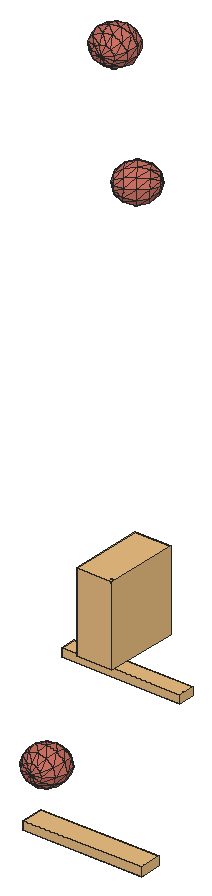
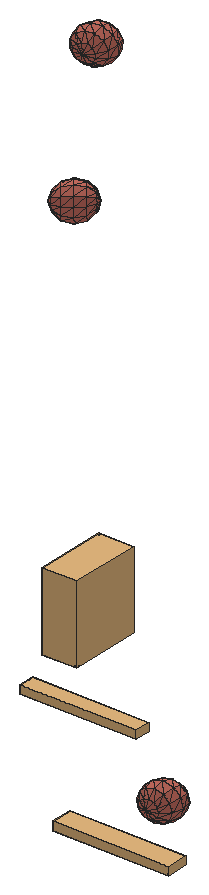
# SketchUp Ruby script. Lengths in inches.
U = 1.inch
M = Sketchup.active_model
def pt(a) = Geom::Point3d.new(a.map { |v| v * U })
def face(e, loops, mat)
  f = e.add_face(loops[0].map { |a| pt(a) })
  loops[1..].each { |l| e.add_face(l.map { |a| pt(a) }).erase! }
  f.material = f.back_material = mat if mat
  f
end
# faces: each face lists its corners as indices into pts; further lists are holes
def faces(e, pts, list, mat = nil) = list.each { |f| face(e, (f[0].is_a?(Array) ? f : [f]).map { |l| l.map { |i| pts[i] } }, mat) }
# xy, xz, yz: faces in a plane at the given z, y or x. An outline is a flat list of corners, or four numbers for a rectangle; further outlines are holes
def ring(l) = l.size == 4 ? [[l[0], l[1]], [l[2], l[1]], [l[2], l[3]], [l[0], l[3]]] : l.each_slice(2).to_a
def flat(e, list, mat, &to3) = list.each { |f| face(e, (f[0].is_a?(Array) ? f : [f]).map { |l| ring(l).map { |u, v| to3.(u, v) } }, mat) }
def xy(e, z, list, mat = nil) = flat(e, list, mat) { |x, y| [x, y, z] }
def xz(e, y, list, mat = nil) = flat(e, list, mat) { |x, z| [x, y, z] }
def yz(e, x, list, mat = nil) = flat(e, list, mat) { |y, z| [x, y, z] }
def lines(e, pts, list) = list.each { |a, b| e.add_line(pt(pts[a]), pt(pts[b])) }
# prism: a flat outline (further loops are holes) pulled along v
def prism(e, loops, v, mat = nil)
  f = face(e, loops, mat); d = Geom::Vector3d.new(v.map { |x| x * U })
  f.pushpull(f.normal.samedirection?(d) ? d.length : -d.length)
end
def box(e, o, s, mat = nil) = prism(e, [[o, [o[0] + s[0], o[1], o[2]], [o[0] + s[0], o[1] + s[1], o[2]], [o[0], o[1] + s[1], o[2]]]], [0, 0, s[2]], mat)
def at(x, y, z, deg = 0) = Geom::Transformation.translation(pt([x, y, z])) * Geom::Transformation.rotation(ORIGIN, Z_AXIS, deg.degrees)
def axes(o, x, y, z) = Geom::Transformation.new([*x, 0, *y, 0, *z, 0, *pt(o).to_a, 1])
def part(name) = M.definitions.add(name)
# library, detail: a bought-in or finely detailed component or shape, given as its bounding box
def library(name, o, s) = part(name).tap { |d| box(d.entities, o, s) }
def detail(e, o, s) = box(e.add_group.entities, o, s)
def put(e, d, t, mat = nil) = e.add_instance(d, t).tap { |i| i.material = mat if mat }
def group(e, t, mat = nil) = e.add_group.tap { |g| g.transformation = t; g.material = mat if mat }.entities
root = M.entities
M.materials.add("green").color = [174, 139, 102]
M.materials.add("vio").color = [206, 114, 100]
c1 = library("3DGeom~15_Defintion",[-93.43,-35.39,-500],[186.86,70.78,1000])
c2 = part("3DGeom~16_Defintion")
p = [[-67.78,-34.5625,-497.5],[-75.6,-25.33,-500],[-54.89,-33.15,-493.42],[-75.6,-25.33,-500],[-67.78,-34.5625,-497.5],[-73.08,-30.88,-499.18],
  [-54.89,-33.15,-493.42],[-75.6,-25.33,-500],[-49.81,-22.5,-491.85],[-75.6,-25.33,-500],[-74.66,-19.4,-499.72],[-70.52,-14.68,-498.43],
  [-57.625,-13.26,-494.36],[-75.6,-25.33,-500],[-70.52,-14.68,-498.43],[-49.81,-22.5,-491.85],[-75.6,-25.33,-500],[-57.625,-13.26,-494.36],
  [-57.625,-13.26,-494.36],[-70.52,-14.68,-498.43],[-64.28,-12.43,-496.47],[-67.78,-34.5625,-497.5],[-54.89,-33.15,-493.42],[-61.125,-35.39,-495.39],
  [-49.81,-22.5,-491.85],[-57.625,-13.26,-494.36],[-52.33,-16.95,-492.67],[-54.89,-33.15,-493.42],[-49.81,-22.5,-491.85],[-50.75,-28.42,-492.13],
  [67.2,22.73,500],[92.46,19.2,493.88],[93.43,25.1,493.15],[67.2,22.73,500],[93.43,25.1,493.15],[90.88,30.68,493.34],
  [67.2,22.73,500],[90.88,30.68,493.34],[85.51,34.45,494.39],[67.2,22.73,500],[88.24,14.5625,495.33],[92.46,19.2,493.88],
  [67.2,22.73,500],[85.51,34.45,494.39],[78.74,35.39,496.03],[67.2,22.73,500],[81.9,12.43,497.11],[88.24,14.5625,495.33],
  [67.2,22.73,500],[78.74,35.39,496.03],[72.39,33.26,497.82],[67.2,22.73,500],[75.13,13.38,498.76],[81.9,12.43,497.11],
  [67.2,22.73,500],[72.39,33.26,497.82],[68.17,28.625,499.27],[67.2,22.73,500],[69.75,17.15,499.8125],[75.13,13.38,498.76]]
faces(c2.entities,p,[[0,1,2],[3,4,5],[6,7,8],[9,10,11],[12,13,14],[15,16,17],[18,19,20],[21,22,23],
  [24,25,26],[27,28,29],[30,31,32],[33,34,35],[36,37,38],[39,40,41],[42,43,44],[45,46,47],
  [48,49,50],[51,52,53],[54,55,56],[57,58,59]],"green")
c3 = part("3DGeom~188_Defintion")
p = [[-5.63,-212.24,-433.01],[-255.63,0,-429.76],[-6.51,0,-500],[245.12,-183.8,-378.25],[244.37,0,-436.27],[-254.88,183.8,-371.75],
  [-5.63,212.24,-433.01],[430.2,-106.12,-222.14],[430.2,-106.12,-222.14],[429.76,0,-255.63],[245.12,183.8,-378.25],[429.76,0,-255.63],
  [245.12,183.8,-378.25],[-3.25,-367.61,-250],[-254.88,-183.8,-371.75],[247.18,-318.36,-219.76],[247.18,-318.36,-219.76],[-252.82,318.36,-213.25],
  [245.12,183.8,-378.25],[-3.25,367.61,-250],[-252.82,318.36,-213.25],[-3.25,367.61,-250],[-254.88,-183.8,-371.75],[-436.27,0,-244.37],
  [-255.63,0,-429.76],[-255.63,0,-429.76],[-435.83,106.12,-210.87],[-255.63,0,-429.76],[-254.88,183.8,-371.75],[431.39,-183.8,-130.63],
  [247.18,-318.36,-219.76],[245.12,-183.8,-378.25],[245.12,-183.8,-378.25],[430.2,-106.12,-222.14],[429.76,0,-255.63],[245.12,183.8,-378.25],
  [430.2,106.12,-222.14],[430.2,106.12,-222.14],[245.12,183.8,-378.25],[247.18,318.36,-219.76],[245.12,183.8,-378.25],[-3.25,367.61,-250],
  [247.18,318.36,-219.76],[-252.82,-318.36,-213.25],[-252.82,-318.36,-213.25],[-435.83,-106.12,-210.87],[-254.88,-183.8,-371.75],[-254.88,-183.8,-371.75],
  [-254.88,183.8,-371.75],[-434.64,183.8,-119.36],[-254.88,183.8,-371.75],[-252.82,318.36,-213.25],[429.76,0,-255.63],[500,0,-6.51],
  [0,-424.48,0],[-252.82,-318.36,-213.25],[-3.25,-367.61,-250],[250,-367.61,-3.25],[-3.25,-367.61,-250],[250,-367.61,-3.25],
  [-3.25,-367.61,-250],[247.18,-318.36,-219.76],[-3.25,367.61,-250],[-252.82,318.36,-213.25],[-250,367.61,3.25],[247.18,318.36,-219.76],
  [0,424.48,0],[-500,0,6.51],[431.39,183.8,-130.63],[433.01,-212.24,-5.63],[250,-367.61,-3.25],[250,367.61,-3.25],
  [247.18,318.36,-219.76],[250,367.61,-3.25],[-250,-367.61,3.25],[-252.82,-318.36,-213.25],[-250,-367.61,3.25],[-434.64,-183.8,-119.37],
  [-252.82,-318.36,-213.25],[-252.82,-318.36,-213.25],[-252.82,318.36,-213.25],[-433.01,212.24,5.63],[-252.82,318.36,-213.25],[-250,367.61,3.25],
  [433.01,212.24,-5.63],[-250,-367.61,3.25],[-433.01,-212.24,5.63],[434.64,-183.8,119.37],[435.83,-106.12,210.87],[436.27,0,244.37],
  [434.64,183.8,119.37],[435.83,106.12,210.87],[252.82,318.36,213.25],[252.82,-318.36,213.25],[250,-367.61,-3.25],[252.82,-318.36,213.25],
  [250,367.61,-3.25],[3.25,367.61,250],[252.82,318.36,213.25],[250,367.61,-3.25],[3.25,367.61,250],[3.25,-367.61,250],
  [252.82,-318.36,213.25],[-247.18,318.36,219.76],[-247.18,318.36,219.76],[3.25,367.61,250],[-247.18,-318.36,219.76],[-250,-367.61,3.25],
  [-247.18,-318.36,219.76],[-250,367.61,3.25],[-431.39,183.8,130.63],[-250,367.61,3.25],[-247.18,318.36,219.76],[-247.18,-318.36,219.76],
  [-431.39,-183.8,130.63],[-430.2,-106.12,222.14],[-429.76,0,255.63],[-429.76,0,255.63],[-430.2,106.12,222.14],[-430.2,106.12,222.14],
  [254.88,183.8,371.75],[-245.12,-183.8,378.25],[-247.18,-318.36,219.76],[-245.12,-183.8,378.25],[-247.18,318.36,219.76],[-430.2,106.12,222.14],
  [254.88,-183.8,371.75],[255.63,0,429.76],[254.88,-183.8,371.75],[3.25,-367.61,250],[252.82,-318.36,213.25],[252.82,318.36,213.25],
  [5.63,212.24,433.01],[254.88,183.8,371.75],[252.82,318.36,213.25],[3.25,367.61,250],[5.63,-212.24,433.01],[-247.18,-318.36,219.76],
  [3.25,-367.61,250],[-245.12,-183.8,378.25],[-247.18,-318.36,219.76],[-247.18,318.36,219.76],[-430.2,106.12,222.14],[-245.12,183.8,378.25],
  [-247.18,318.36,219.76],[-245.12,183.8,378.25],[-244.37,0,436.27],[-430.2,-106.12,222.14],[-429.76,0,255.63],[-430.2,-106.12,222.14],
  [-430.2,106.12,222.14],[254.88,-183.8,371.75],[3.25,-367.61,250],[255.63,0,429.76],[254.88,-183.8,371.75],[254.88,183.8,371.75],
  [6.51,0,500],[254.88,183.8,371.75],[255.63,0,429.76],[255.63,0,429.76]]
faces(c3.entities,p,[[0,1,2],[3,0,2],[3,2,4],[2,1,5],[2,5,6],[4,2,6],[7,3,4],[8,4,9],
  [4,6,10],[11,4,12],[13,14,0],[15,13,0],[16,0,3],[0,14,1],[6,5,17],[18,6,19],
  [6,20,21],[22,23,24],[25,23,26],[27,26,28],[29,30,31],[29,32,33],[34,35,36],[37,38,39],
  [40,41,42],[13,43,14],[44,45,46],[47,45,23],[48,26,49],[50,49,51],[33,52,53],[52,37,53],
  [54,55,56],[57,54,58],[59,60,61],[62,63,64],[65,62,66],[62,64,66],[23,45,67],[26,23,67],
  [29,33,53],[37,68,53],[37,39,68],[69,70,30],[69,30,29],[68,39,71],[72,66,73],[54,74,75],
  [76,77,78],[79,77,45],[80,49,81],[82,81,83],[45,77,67],[49,26,67],[69,29,53],[68,84,53],
  [68,71,84],[85,86,77],[77,86,67],[81,49,67],[87,69,53],[88,87,53],[89,88,53],[84,90,53],
  [90,91,53],[91,89,53],[87,70,69],[84,92,90],[84,71,92],[93,54,94],[87,95,70],[96,97,98],
  [99,66,100],[101,74,54],[102,101,54],[66,64,103],[66,104,105],[106,86,107],[101,108,74],[109,81,110],
  [111,110,112],[113,114,86],[86,114,67],[110,81,67],[114,115,67],[115,116,67],[117,118,67],[119,110,67],
  [88,95,87],[90,120,91],[90,92,120],[121,114,122],[123,115,114],[124,110,125],[88,126,95],[89,126,88],
  [91,120,127],[91,127,89],[128,129,130],[131,132,133],[134,135,132],[136,137,138],[136,139,140],[141,142,143],
  [135,144,145],[146,147,139],[146,148,149],[145,150,148],[89,127,126],[151,136,152],[135,145,132],[145,148,146],
  [153,136,154],[155,132,156],[157,156,158],[156,139,136],[156,146,139],[132,145,146],[159,156,136],[132,146,156]],"vio")
c4 = part("3DGeom~198_Defintion")
p = [[-186.75,95.89,-455.78],[73.04,104.68,-484.59],[66.15,-117.28,-481.5625],[307.29,-106.8,-380.93],[313.25,85.42,-383.56],[60.35,298.59,-357.77],
  [-197.73,263.82,-345.95],[-192.71,-96.34,-453.16],[41.54,-307.82,-349.5],[285.98,-271.8125,-266.57],[-396.49,61.4,-304.84],[-402.84,158.36,-241.43],
  [-396.49,61.4,-304.84],[-402.84,158.36,-241.43],[-214.02,-261.34,-338.79],[-399.9375,-49.58,-303.33],[-396.49,61.4,-304.84],[-399.9375,-49.58,-303.33],
  [313.25,85.42,-383.56],[466.09,-67.71,-178.23],[307.29,-106.8,-380.93],[313.25,85.42,-383.56],[469.53,43.27,-179.75],[302.27,253.36,-273.73],
  [313.25,85.42,-383.56],[302.27,253.36,-273.73],[307.29,-106.8,-380.93],[453.78,-162.97,-112.2],[285.98,-271.8125,-266.57],[307.29,-106.8,-380.93],
  [31.5,412.5,-135.08],[302.27,253.36,-273.73],[60.35,298.59,-357.77],[-222.72,362.47,-153.1],[60.35,298.59,-357.77],[-197.73,263.82,-345.95],
  [-222.72,362.47,-153.1],[60.35,298.59,-357.77],[-214.02,-261.34,-338.79],[41.54,-307.82,-349.5],[5.8,-415.875,-123.8],[41.54,-307.82,-349.5],
  [255.02,-365.39,-71.1],[41.54,-307.82,-349.5],[285.98,-271.8125,-266.57],[-417.26,215.3125,-130.09],[-197.73,263.82,-345.95],[-402.84,158.36,-241.43],
  [-222.72,362.47,-153.1],[-197.73,263.82,-345.95],[-214.02,-261.34,-338.79],[-244.98,-354.93,-143.32],[-412.24,-144.85,-237.3],[-214.02,-261.34,-338.79],
  [-244.98,-354.93,-143.32],[-399.9375,-49.58,-303.33],[-412.24,-144.85,-237.3],[-396.49,61.4,-304.84],[-399.9375,-49.58,-303.33],[-500,10.47,-72.22],
  [302.27,253.36,-273.73],[463.1875,140.23,-116.34],[277.28,352,-80.875],[302.27,253.36,-273.73],[277.28,352,-80.875],[302.27,253.36,-273.73],
  [285.98,-271.8125,-266.57],[435.91,-217,0.65],[255.02,-365.39,-71.1],[285.98,-271.8125,-266.57],[-430.11,-198.87,-124.44],[500,-10.47,72.22],
  [-435.91,217,-0.65],[-255.02,365.39,71.1],[-255.02,365.39,71.1],[-222.72,362.47,-153.1],[-244.98,-354.93,-143.32],[-31.5,-412.49,135.08],
  [-244.98,-354.93,-143.32],[-277.28,-352,80.875],[-277.28,-352,80.875],[-5.8,415.875,123.8],[-255.02,365.39,71.1],[-448.76,-197.18,5],
  [222.72,-362.47,153.1],[448.76,197.18,-4.99],[277.28,352,-80.875],[244.98,354.93,143.32],[277.28,352,-80.875],[244.98,354.93,143.32],
  [-463.1875,-140.23,116.34],[-469.53,-43.27,179.75],[-466.09,67.71,178.23],[-453.78,162.97,112.2],[255.02,-365.39,-71.1],[417.26,-215.3125,130.09],
  [222.72,-362.47,153.1],[255.02,-365.39,-71.1],[430.11,198.87,124.44],[244.98,354.93,143.32],[-302.27,-253.36,273.73],[-285.98,271.8125,266.57],
  [-285.98,271.8125,266.57],[-255.02,365.39,71.1],[402.84,-158.36,241.43],[396.49,-61.4,304.84],[402.84,-158.36,241.43],[399.9375,49.58,303.33],
  [396.49,-61.4,304.84],[412.24,144.85,237.3],[399.9375,49.58,303.33],[-277.28,-352,80.875],[-60.35,-298.59,357.77],[-277.28,-352,80.875],
  [-60.35,-298.59,357.77],[-302.27,-253.36,273.73],[-313.25,-85.42,383.56],[-285.98,271.8125,266.57],[-41.54,307.82,349.5],[214.02,261.34,338.79],
  [214.02,261.34,338.79],[244.98,354.93,143.32],[222.72,-362.47,153.1],[402.84,-158.36,241.43],[197.73,-263.82,345.95],[-60.35,-298.59,357.77],
  [197.73,-263.82,345.95],[214.02,261.34,338.79],[222.72,-362.47,153.1],[402.84,-158.36,241.43],[197.73,-263.82,345.95],[-307.29,106.8,380.93],
  [192.71,96.34,453.16],[399.9375,49.58,303.33],[412.24,144.85,237.3],[412.24,144.85,237.3],[214.02,261.34,338.79],[197.73,-263.82,345.95],
  [402.84,-158.36,241.43],[396.49,-61.4,304.84],[-307.29,106.8,380.93],[-41.54,307.82,349.5],[-285.98,271.8125,266.57],[-302.27,-253.36,273.73],
  [-60.35,-298.59,357.77],[-73.04,-104.68,484.59],[-302.27,-253.36,273.73],[-313.25,-85.42,383.56],[186.75,-95.89,455.78],[-66.15,117.28,481.5625],
  [214.02,261.34,338.79],[214.02,261.34,338.79],[-41.54,307.82,349.5],[-307.29,106.8,380.93],[-41.54,307.82,349.5],[-313.25,-85.42,383.56],
  [-307.29,106.8,380.93],[-313.25,-85.42,383.56]]
faces(c4.entities,p,[[0,1,2],[1,3,2],[1,4,3],[5,4,1],[6,1,0],[6,5,1],[7,2,8],[2,9,8],
  [2,3,9],[0,2,7],[10,0,7],[11,0,12],[13,6,0],[7,8,14],[15,7,14],[16,7,17],
  [18,19,20],[21,22,19],[23,22,24],[5,25,4],[26,27,28],[29,19,27],[30,31,32],[33,34,35],
  [36,30,37],[38,39,40],[41,42,40],[43,44,42],[45,46,47],[45,48,49],[50,40,51],[52,53,54],
  [55,14,56],[57,58,59],[47,57,59],[58,52,59],[60,61,22],[62,61,63],[30,64,65],[66,67,68],
  [69,27,67],[45,47,59],[52,54,70],[52,70,59],[19,22,71],[22,61,71],[27,19,71],[72,48,45],
  [72,73,48],[74,30,75],[76,40,77],[78,77,79],[70,54,80],[81,64,30],[82,81,30],[72,45,59],
  [70,80,83],[70,83,59],[40,84,77],[40,42,84],[61,85,71],[86,85,61],[67,27,71],[87,85,88],
  [81,89,64],[83,90,59],[90,91,59],[91,92,59],[93,72,59],[92,93,59],[94,95,96],[97,67,95],
  [85,98,71],[99,98,85],[93,73,72],[95,67,71],[83,80,100],[83,100,90],[93,101,73],[102,81,103],
  [104,95,71],[105,106,71],[107,108,71],[109,110,71],[98,109,71],[111,77,112],[113,114,115],[92,101,93],
  [90,100,116],[90,116,91],[117,118,81],[118,89,81],[119,109,98],[120,98,121],[122,95,123],[77,124,125],
  [77,84,126],[118,127,89],[128,129,130],[91,131,92],[92,131,101],[91,116,131],[132,133,134],[132,135,136],
  [137,138,139],[140,141,142],[143,144,145],[146,145,147],[148,139,133],[148,133,132],[137,139,148],[149,132,150],
  [149,151,152],[144,137,148],[153,149,154],[144,148,145],[155,149,156],[157,145,149],[145,148,132],[145,132,149]],"vio")
c5 = library("3DGeom~115_Defintion",[-457.23,-500,-223.02],[914.46,1000,446.04])
c6 = part("3DGeom~116_Defintion")
p = [[-442.89,-492.22,-212.42],[-434.63,-497.16,-209.35],[-428.12,-500,-201.74],[-426.4,-497.09,-181.7],[-442.89,-492.22,-212.42],[-428.12,-500,-201.74],
  [-439.45,-486.4,-172.35],[-442.89,-492.22,-212.42],[-426.4,-497.09,-181.7],[-455.93,-481.53,-203.07],[-442.89,-492.22,-212.42],[-454.21,-478.62,-183.03],
  [-442.89,-492.22,-212.42],[-455.93,-481.53,-203.07],[-450.6875,-486.5,-210.125],[-454.21,-478.62,-183.03],[-442.89,-492.22,-212.42],[-439.45,-486.4,-172.35],
  [-455.93,-481.53,-203.07],[-454.21,-478.62,-183.03],[-457.23,-478.65,-193.16],[-426.4,-497.09,-181.7],[-428.12,-500,-201.74],[-425.11,-499.97,-191.61],
  [-454.21,-478.62,-183.03],[-439.45,-486.4,-172.35],[-447.71,-481.46,-175.42],[-439.45,-486.4,-172.35],[-426.4,-497.09,-181.7],[-431.65,-492.12,-174.65],
  [445.89,493.0625,185.04],[444.32,479.16,220.86],[452.08,476.9375,214.19],[445.89,493.0625,185.04],[452.08,476.9375,214.19],[456.81,477.81,204.8],
  [445.89,493.0625,185.04],[456.81,477.81,204.8],[457.23,481.53,195.2],[445.89,493.0625,185.04],[435.6,483.875,223.02],[444.32,479.16,220.86],
  [445.89,493.0625,185.04],[457.23,481.53,195.2],[453.23,487.12,187.97],[445.89,493.0625,185.04],[428.26,489.82,220.09],[435.6,483.875,223.02],
  [445.89,493.0625,185.04],[424.27,495.41,212.85],[428.26,489.82,220.09],[445.89,493.0625,185.04],[424.6875,499.13,203.26],[424.27,495.41,212.85],
  [445.89,493.0625,185.04],[429.41,500,193.87],[424.6875,499.13,203.26],[445.89,493.0625,185.04],[437.17,497.78,187.2],[429.41,500,193.87]]
faces(c6.entities,p,[[0,1,2],[3,4,5],[6,7,8],[9,10,11],[12,13,14],[15,16,17],[18,19,20],[21,22,23],
  [24,25,26],[27,28,29],[30,31,32],[33,34,35],[36,37,38],[39,40,41],[42,43,44],[45,46,47],
  [48,49,50],[51,52,53],[54,55,56],[57,58,59]],"green")
c7 = part("3DGeom~197_Defintion")
p = [[121.86,-140.79,-463.73],[-185.76,-85.76,-461.18],[69.15,-43.45,-500],[305.53,10.51,-404.84],[-186.34,107.23,-454.67],[68.81,67.97,-496.24],
  [305.53,10.51,-404.84],[120.9375,163.62,-453.46],[305.53,10.51,-404.84],[-96.06,272.89,-380.57],[-94.47,-254.36,-398.36],[212.81,-197.97,-397.15],
  [305.53,10.51,-404.84],[-390.89,-105.1,-298.79],[-391.57,117.75,-291.27],[-287.32,309.04,-205.7],[-287.32,309.04,-205.7],[211.56,217.86,-383.12],
  [305.53,10.51,-404.84],[60.9,366.84,-258.73],[60.9,366.84,-258.73],[317.64,-199.66,-318.1],[305.53,10.51,-404.84],[408.26,-145.42,-247.75],
  [305.53,10.51,-404.84],[460.38,-49.77,-204.97],[408.26,-145.42,-247.75],[305.53,10.51,-404.84],[460.04,61.65,-201.21],[316.39,216.17,-304.0625],
  [305.53,10.51,-404.84],[407.34,158.99,-237.48],[316.39,216.17,-304.0625],[63.06,-353.4,-283.04],[-285.48,-299.78,-226.25],[-94.47,-254.36,-398.36],
  [63.06,-353.4,-283.04],[-285.48,-299.78,-226.25],[317.64,-199.66,-318.1],[63.06,-353.4,-283.04],[212.81,-197.97,-397.15],[211.56,217.86,-383.12],
  [242.47,363.91,-121.81],[316.39,216.17,-304.0625],[211.56,217.86,-383.12],[60.9,366.84,-258.73],[242.47,363.91,-121.81],[-96.06,272.89,-380.57],
  [-287.32,309.04,-205.7],[-106.08,417.53,-65.02],[-96.06,272.89,-380.57],[317.64,-199.66,-318.1],[244.64,-356.33,-146.11],[63.06,-353.4,-283.04],
  [244.64,-356.33,-146.11],[317.64,-199.66,-318.1],[400,264.87,-6.48],[242.47,363.91,-121.81],[-285.48,-299.78,-226.25],[-491.29,-96.27,-56.34],
  [-390.89,-105.1,-298.79],[-390.89,-105.1,-298.79],[-491.87,96.72,-49.82],[-390.89,-105.1,-298.79],[-391.57,117.75,-291.27],[-391.57,117.75,-291.27],
  [-401.59,262.38,24.28],[-391.57,117.75,-291.27],[-401.59,262.38,24.28],[-287.32,309.04,-205.7],[63.06,-353.4,-283.04],[-103.58,-414.14,-93.09],
  [-285.48,-299.78,-226.25],[63.06,-353.4,-283.04],[103.58,414.14,93.09],[242.47,363.91,-121.81],[401.59,-262.38,-24.28],[244.64,-356.33,-146.11],
  [491.29,96.27,56.34],[-400,-264.87,6.48],[-285.48,-299.78,-226.25],[-285.48,-299.78,-226.25],[-400,-264.87,6.48],[-401.59,262.38,24.28],
  [-244.64,356.33,146.11],[491.87,-96.72,49.82],[106.08,-417.53,65.02],[401.59,-262.38,-24.28],[242.47,363.91,-121.81],[285.48,299.78,226.25],
  [400,264.87,-6.48],[242.47,363.91,-121.81],[285.48,299.78,226.25],[-242.47,-363.91,121.81],[-400,-264.87,6.48],[-63.06,353.4,283.04],
  [-460.04,-61.65,201.21],[-460.38,49.77,204.97],[-408.26,145.42,247.75],[-401.59,262.38,24.28],[401.59,-262.38,-24.28],[287.32,-309.04,205.7],
  [287.32,-309.04,205.7],[390.89,105.1,298.79],[285.48,299.78,226.25],[-242.47,-363.91,121.81],[-407.34,-158.99,237.48],[-401.59,262.38,24.28],
  [-317.64,199.66,318.1],[-401.59,262.38,24.28],[-317.64,199.66,318.1],[-244.64,356.33,146.11],[391.57,-117.75,291.27],[-60.9,-366.84,258.73],
  [287.32,-309.04,205.7],[94.47,254.36,398.36],[94.47,254.36,398.36],[285.48,299.78,226.25],[-316.39,-216.17,304.0625],[-242.47,-363.91,121.81],
  [-316.39,-216.17,304.0625],[-317.64,199.66,318.1],[-212.81,197.97,397.15],[-212.81,197.97,397.15],[-305.53,-10.51,404.84],[-305.53,-10.51,404.84],
  [-305.53,-10.51,404.84],[287.32,-309.04,205.7],[96.06,-272.89,380.57],[391.57,-117.75,291.27],[96.06,-272.89,380.57],[287.32,-309.04,205.7],
  [285.48,299.78,226.25],[94.47,254.36,398.36],[185.76,85.76,461.18],[285.48,299.78,226.25],[390.89,105.1,298.79],[-305.53,-10.51,404.84],
  [-317.64,199.66,318.1],[-408.26,145.42,247.75],[-305.53,-10.51,404.84],[-211.56,-217.86,383.11],[-316.39,-216.17,304.0625],[-211.56,-217.86,383.11],
  [-60.9,-366.84,258.73],[-63.06,353.4,283.04],[-212.81,197.97,397.15],[-121.86,140.79,463.73],[-63.06,353.4,283.04],[391.57,-117.75,291.27],
  [186.34,-107.23,454.67],[390.89,105.1,298.79],[391.57,-117.75,291.27],[390.89,105.1,298.79],[-316.39,-216.17,304.0625],[-211.56,-217.86,383.11],
  [-317.64,199.66,318.1],[-120.9375,-163.62,453.46],[-211.56,-217.86,383.11],[-211.56,-217.86,383.11],[-69.15,43.45,500],[-68.81,-67.97,496.24]]
faces(c7.entities,p,[[0,1,2],[0,2,3],[2,1,4],[2,4,5],[2,5,6],[5,7,8],[5,4,9],[5,9,7],
  [0,10,1],[11,10,0],[11,0,12],[10,13,1],[1,13,14],[1,14,4],[4,14,15],[4,16,9],
  [7,17,18],[7,9,19],[7,20,17],[21,11,22],[23,21,24],[25,26,27],[28,25,27],[17,29,30],
  [31,28,27],[32,31,27],[33,34,35],[11,36,10],[10,37,13],[38,39,40],[41,42,43],[44,45,46],
  [47,48,49],[50,49,45],[51,52,53],[26,54,55],[32,56,31],[32,57,56],[58,59,60],[61,59,62],
  [63,62,64],[65,62,66],[67,68,69],[70,71,72],[52,71,73],[45,74,75],[45,49,74],[26,76,77],
  [25,76,26],[31,78,28],[31,56,78],[71,79,80],[81,82,59],[48,83,84],[48,84,49],[25,85,76],
  [28,85,25],[28,78,85],[52,86,71],[87,86,52],[88,89,90],[91,74,92],[86,93,71],[71,93,94],
  [49,84,95],[49,95,74],[82,96,59],[59,97,62],[59,96,97],[62,97,98],[62,98,99],[100,101,86],
  [85,102,76],[56,103,78],[56,104,103],[105,106,82],[82,106,96],[107,98,108],[109,110,111],[85,112,102],
  [78,112,85],[78,103,112],[86,113,93],[114,113,86],[74,95,115],[74,116,117],[113,118,93],[119,120,106],
  [84,121,122],[84,123,95],[96,106,124],[97,96,125],[98,97,126],[127,128,113],[129,130,131],[132,133,134],
  [135,134,136],[106,120,137],[138,139,140],[113,141,142],[130,143,144],[145,146,147],[148,147,133],[149,150,130],
  [151,150,152],[153,134,150],[154,155,140],[146,156,140],[130,157,158],[150,157,130],[159,157,140],[147,146,140],
  [133,147,160],[133,160,134],[157,161,140],[161,160,140],[160,147,140],[150,161,157],[134,161,150],[134,160,161]],"vio")
c8 = library("3DGeom~117_Defintion",[-67.35,-35.15,-500],[134.7,70.3,1000])
c9 = part("3DGeom~118_Defintion")
p = [[-32.48,-34.33,-497.04],[-40.08,-25.16,-500],[-19.94,-32.92,-492.22],[-40.08,-25.16,-500],[-32.48,-34.33,-497.04],[-37.63,-30.67,-499.04],
  [-19.94,-32.92,-492.22],[-40.08,-25.16,-500],[-15,-22.34,-490.36],[-40.08,-25.16,-500],[-39.16,-19.27,-499.67],[-35.13,-14.58,-498.14],
  [-22.6,-13.17,-493.32],[-40.08,-25.16,-500],[-35.13,-14.58,-498.14],[-15,-22.34,-490.36],[-40.08,-25.16,-500],[-22.6,-13.17,-493.32],
  [-22.6,-13.17,-493.32],[-35.13,-14.58,-498.14],[-29.07,-12.35,-495.8125],[-32.48,-34.33,-497.04],[-19.94,-32.92,-492.22],[-26.01,-35.15,-494.55],
  [-15,-22.34,-490.36],[-22.6,-13.17,-493.32],[-17.45,-16.83,-491.32],[-19.94,-32.92,-492.22],[-15,-22.34,-490.36],[-15.92,-28.23,-490.69],
  [40.93,22.57,500],[66.34,19.07,495.46],[67.35,24.92,494.8],[40.93,22.57,500],[64.81,30.47,494.83],[59.41,34.21,495.55],
  [40.93,22.57,500],[67.35,24.92,494.8],[64.81,30.47,494.83],[40.93,22.57,500],[62.07,14.46,496.64],[66.34,19.07,495.46],
  [40.93,22.57,500],[59.41,34.21,495.55],[52.61,35.15,496.77],[40.93,22.57,500],[55.67,12.35,498.03],[62.07,14.46,496.64],
  [40.93,22.57,500],[52.61,35.15,496.77],[46.21,33.04,498.15],[40.93,22.57,500],[48.86,13.29,499.25],[55.67,12.35,498.03],
  [40.93,22.57,500],[46.21,33.04,498.15],[41.93,28.43,499.34],[40.93,22.57,500],[43.47,17.03,499.97],[48.86,13.29,499.25]]
faces(c9.entities,p,[[0,1,2],[3,4,5],[6,7,8],[9,10,11],[12,13,14],[15,16,17],[18,19,20],[21,22,23],
  [24,25,26],[27,28,29],[30,31,32],[33,34,35],[36,37,38],[39,40,41],[42,43,44],[45,46,47],
  [48,49,50],[51,52,53],[54,55,56],[57,58,59]],"green")
g1 = group(root,at(15.3125,134.49,26.21))
put(g1,c1,axes([2.99,0.13,10.6],[0,0.00109,0],[0,0,-0.00109],[-0.00109,0,0]),"green")
put(g1,c2,axes([2.99,0.13,10.6],[0,0.00109,0],[0,0,-0.00109],[-0.00109,0,0]),"green")
g2 = group(root,at(15.3125,134.49,26.21))
put(g2,c3,axes([2.58,0.13,11.1],[0,0.00039,0],[0,0,-0.00039],[-0.00039,0,0]),"vio")
g3 = group(root,at(15.3125,134.49,26.21))
put(g3,c4,axes([3.21,0.13,17.26],[0,0.00039,0],[0,0,-0.00039],[-0.00039,0,0]),"vio")
g4 = group(root,at(15.3125,134.49,26.21))
put(g4,c5,axes([3.2,0.24,12.62],[0,0.00073,0],[0,0,-0.00073],[-0.00073,0,0]),"green")
put(g4,c6,axes([3.2,0.24,12.62],[0,0.00073,0],[0,0,-0.00073],[-0.00073,0,0]),"green")
g5 = group(root,at(15.3125,134.49,26.21))
put(g5,c7,axes([3.23,0.36,16.03],[0,0.00038,0],[0,0,-0.00038],[-0.00038,0,0]),"vio")
g6 = group(root,at(15.3125,134.49,26.21))
put(g6,c8,axes([3.04,0.48,11.875],[0,0.00109,0],[0,0,-0.00109],[-0.00109,0,0]),"green")
put(g6,c9,axes([3.04,0.48,11.875],[0,0.00109,0],[0,0,-0.00109],[-0.00109,0,0]),"green")
